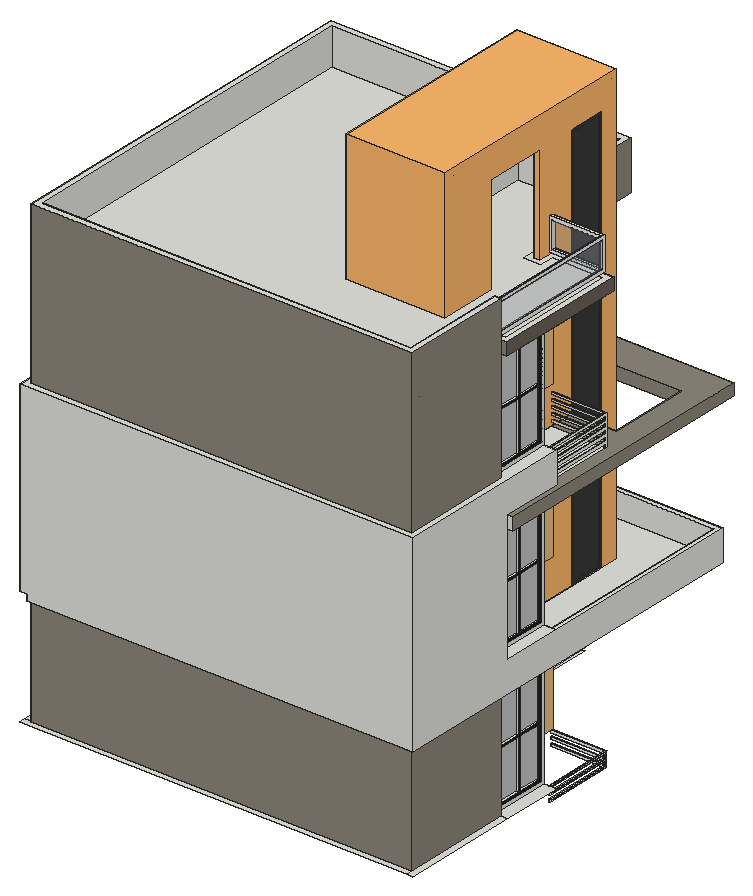
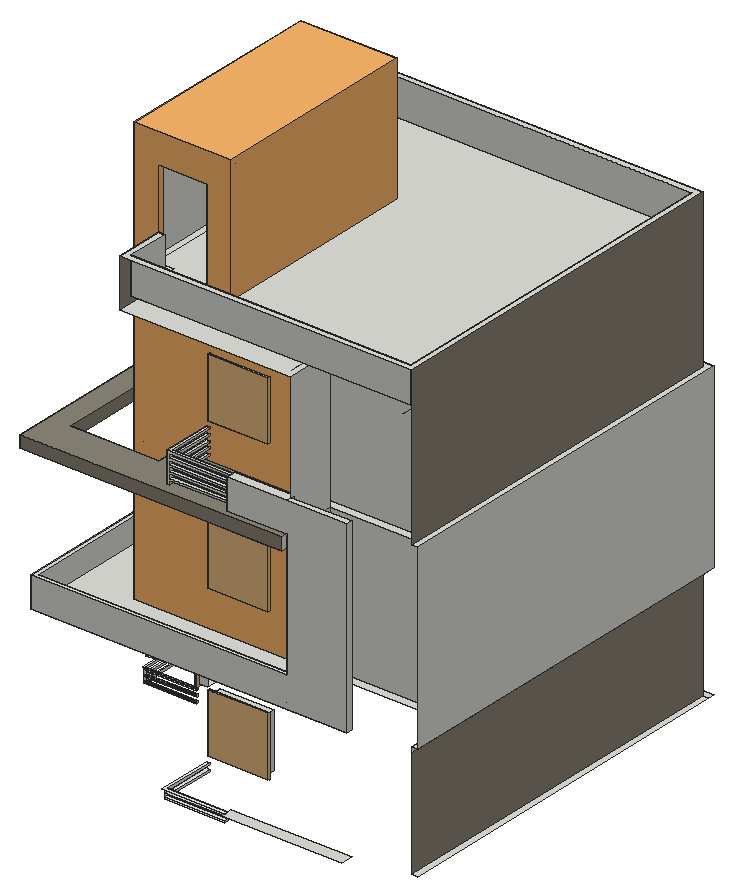
# SketchUp Ruby script. Lengths in inches.
U = 1.inch
M = Sketchup.active_model
def pt(a) = Geom::Point3d.new(a.map { |v| v * U })
def face(e, loops, mat)
  f = e.add_face(loops[0].map { |a| pt(a) })
  loops[1..].each { |l| e.add_face(l.map { |a| pt(a) }).erase! }
  f.material = f.back_material = mat if mat
  f
end
# faces: each face lists its corners as indices into pts; further lists are holes
def faces(e, pts, list, mat = nil) = list.each { |f| face(e, (f[0].is_a?(Array) ? f : [f]).map { |l| l.map { |i| pts[i] } }, mat) }
# xy, xz, yz: faces in a plane at the given z, y or x. An outline is a flat list of corners, or four numbers for a rectangle; further outlines are holes
def ring(l) = l.size == 4 ? [[l[0], l[1]], [l[2], l[1]], [l[2], l[3]], [l[0], l[3]]] : l.each_slice(2).to_a
def flat(e, list, mat, &to3) = list.each { |f| face(e, (f[0].is_a?(Array) ? f : [f]).map { |l| ring(l).map { |u, v| to3.(u, v) } }, mat) }
def xy(e, z, list, mat = nil) = flat(e, list, mat) { |x, y| [x, y, z] }
def xz(e, y, list, mat = nil) = flat(e, list, mat) { |x, z| [x, y, z] }
def yz(e, x, list, mat = nil) = flat(e, list, mat) { |y, z| [x, y, z] }
def lines(e, pts, list) = list.each { |a, b| e.add_line(pt(pts[a]), pt(pts[b])) }
# prism: a flat outline (further loops are holes) pulled along v
def prism(e, loops, v, mat = nil)
  f = face(e, loops, mat); d = Geom::Vector3d.new(v.map { |x| x * U })
  f.pushpull(f.normal.samedirection?(d) ? d.length : -d.length)
end
def box(e, o, s, mat = nil) = prism(e, [[o, [o[0] + s[0], o[1], o[2]], [o[0] + s[0], o[1] + s[1], o[2]], [o[0], o[1] + s[1], o[2]]]], [0, 0, s[2]], mat)
def at(x, y, z, deg = 0) = Geom::Transformation.translation(pt([x, y, z])) * Geom::Transformation.rotation(ORIGIN, Z_AXIS, deg.degrees)
def axes(o, x, y, z) = Geom::Transformation.new([*x, 0, *y, 0, *z, 0, *pt(o).to_a, 1])
def part(name) = M.definitions.add(name)
# library, detail: a bought-in or finely detailed component or shape, given as its bounding box
def library(name, o, s) = part(name).tap { |d| box(d.entities, o, s) }
def detail(e, o, s) = box(e.add_group.entities, o, s)
def put(e, d, t, mat = nil) = e.add_instance(d, t).tap { |i| i.material = mat if mat }
def group(e, t, mat = nil) = e.add_group.tap { |g| g.transformation = t; g.material = mat if mat }.entities
root = M.entities
M.materials.add("Brick_05_1K").color = [255, 185, 107]
M.materials.add("Glass_Basic_01").color = [161, 173, 186]
M.materials["Glass_Basic_01"].alpha = 0.25
M.materials.add("M02_Ash_Whisper").color = [196, 196, 196]
M.materials.add("M07_Charcoal_Gleam").color = [58, 58, 58]
M.materials.add("M08_Obsidian_Black").color = [30, 30, 30]
M.materials.add("Metal_06_1K").color = [238, 236, 231]
M.materials.add("Plaster_04_1K").color = [106, 98, 87]
M.materials.add("Plaster_06_1K").color = [141, 135, 122]
c1 = library("mesh-164",[-1582.71,-3144.16,-23.22],[2366.42,2227.34,65.81])
c2 = part("Group13")
put(c2.entities,c1,at(294.66,859.51,3.5))
xy(root,334,[[491.43,250.15,492.93,317.65],[438.93,317.65,491.43,319.15],[363.93,397.15,366.93,449.15],[303.93,449.15,363.93,453.15]])
xy(root,336,[[491.43,250.15,492.93,317.65],[438.93,317.65,491.43,319.15],[363.93,397.15,366.93,449.15],[303.93,449.15,363.93,453.15]],"Metal_06_1K")
xy(root,340,[[491.43,250.15,492.93,317.65],[438.93,317.65,491.43,319.15],[363.93,397.15,366.93,449.15],[303.93,449.15,363.93,453.15]])
xy(root,342,[[183.93,445.15,303.93,457.15]])
xy(root,342,[[491.43,250.15,492.93,317.65],[438.93,317.65,491.43,319.15],[363.93,397.15,366.93,397.15,366.93,453.15,303.93,453.15,303.93,449.15,363.93,449.15]],"Metal_06_1K")
xy(root,346,[[491.43,250.15,492.93,317.65],[438.93,317.65,491.43,319.15]])
xy(root,348,[[117.93,76.15,492.93,82.15],[492.93,76.15,498.93,190.15],[117.93,82.15,123.93,445.15],[482.43,190.15,486.93,250.15],[486.93,190.15,498.93,250.15]])
xy(root,348,[[491.43,250.15,492.93,250.15,492.93,319.15,438.93,319.15,438.93,317.65,491.43,317.65]],"Metal_06_1K")
xy(root,351,[[429.93,262.15,438.93,316.15],[306.93,388.15,360.93,397.15]])
xy(root,354,[[484.46,196.15,486.93,219.15],[484.46,221.15,486.93,244.15]])
xy(root,402,[[484.46,196.15,486.93,219.15],[484.46,221.15,486.93,244.15]])
xy(root,404,[[484.46,196.15,486.93,219.15],[484.46,221.15,486.93,244.15]])
xy(root,405,[[429.93,262.15,438.93,316.15],[429.93,346.15,438.93,382.15],[306.93,388.15,360.93,397.15]])
xy(root,450,[[484.46,196.15,486.93,219.15],[484.46,221.15,486.93,244.15]])
xy(root,456,[[123.93,76.15,132.93,82.15],[132.93,76.15,429.93,82.15],[492.93,76.15,492.93,190.15,486.93,190.15,486.93,250.15,482.43,250.15,482.43,190.15,438.93,190.15,438.93,397.15,243.93,397.15,243.93,445.15,183.93,445.15,183.93,451.15,498.93,451.15,498.93,76.15],[429.93,76.15,486.93,82.15],[486.93,76.15,492.93,82.15],
  [123.93,82.15,132.93,388.15],[132.93,82.15,429.93,91.15],[429.93,82.15,486.93,82.15,486.93,190.15,438.93,190.15,438.93,388.15,429.93,388.15],[486.93,82.15,492.93,190.15],[132.93,91.15,429.93,388.15]])
xy(root,462,[[117.93,76.15,123.93,445.15],[132.93,91.15,429.93,388.15],[438.93,190.15,482.43,190.15,482.43,250.15,494.43,250.15,494.43,446.65,243.93,446.65,243.93,397.15,438.93,397.15]])
xy(root,464,[[436.93,345.15,438.93,373.15],[436.93,373.15,438.93,377.15]],"M07_Charcoal_Gleam")
xy(root,486,[[482.43,190.15,486.93,250.15],[486.93,190.15,498.93,250.15],[494.43,250.15,498.93,250.15,498.93,451.15,243.93,451.15,243.93,446.65,494.43,446.65]])
xy(root,492,[[484.46,196.15,486.93,219.15],[484.46,221.15,486.93,244.15]])
xy(root,501,[[429.93,262.15,438.93,316.15],[306.93,388.15,360.93,397.15]])
xy(root,543,[[484.46,196.15,486.93,219.15],[484.46,221.15,486.93,244.15]])
xy(root,545,[[484.46,196.15,486.93,219.15],[484.46,221.15,486.93,244.15]])
xy(root,555,[[429.93,262.15,438.93,316.15],[306.93,388.15,360.93,397.15]])
xy(root,594,[[484.46,196.15,486.93,219.15],[484.46,221.15,486.93,244.15]])
xy(root,600,[[438.93,190.15,438.93,343.15,482.43,343.15,482.43,421.55,394.65,421.55,394.65,397.15,243.93,397.15,243.93,457.15,504.93,457.15,504.93,190.15,486.93,190.15,486.93,250.15,482.43,250.15,482.43,190.15]],"Plaster_06_1K")
xy(root,606,[[132.93,91.15,429.93,388.15]])
xy(root,612,[[132.93,91.15,429.93,388.15],[438.93,190.15,482.43,190.15,482.43,250.15,491.43,250.15,491.43,317.65,438.93,317.65],[486.93,190.15,498.93,250.15],[491.43,317.65,492.93,319.15],[243.93,440.65,303.93,451.15]])
xy(root,612,[[498.93,190.15,504.93,190.15,504.93,457.15,243.93,457.15,243.93,451.15,303.93,451.15,303.93,440.65,243.93,440.65,243.93,397.15,394.65,397.15,394.65,421.55,482.43,421.55,482.43,343.15,438.93,343.15,438.93,317.65,491.43,317.65,491.43,319.15,492.93,319.15,492.93,317.65,491.43,317.65,491.43,250.15,498.93,250.15]],"Plaster_06_1K")
xy(root,616,[[491.43,250.15,492.93,317.65],[438.93,317.65,491.43,319.15]])
xy(root,618,[[491.43,250.15,492.93,317.65],[438.93,317.65,491.43,319.15],[363.93,391.1,366.93,397.15],[363.93,397.15,366.93,443.15],[303.93,443.15,363.93,447.15]])
xy(root,622,[[491.43,250.15,492.93,317.65],[438.93,317.65,491.43,319.15]])
xy(root,624,[[491.43,250.15,492.93,317.65],[438.93,317.65,491.43,319.15],[363.93,391.1,366.93,397.15],[363.93,397.15,366.93,443.15],[303.93,443.15,363.93,447.15]])
xy(root,628,[[491.43,250.15,492.93,317.65],[438.93,317.65,491.43,319.15]])
xy(root,630,[[491.43,250.15,492.93,317.65],[438.93,317.65,491.43,319.15],[363.93,391.1,366.93,397.15],[363.93,397.15,366.93,443.15],[303.93,443.15,363.93,447.15]])
xy(root,634,[[491.43,250.15,492.93,317.65],[438.93,317.65,491.43,319.15]])
xy(root,636,[[491.43,250.15,492.93,317.65],[438.93,317.65,491.43,319.15],[363.93,391.15,366.93,397.15],[363.93,397.15,366.93,443.15],[303.93,443.15,363.93,447.15]])
xy(root,640,[[491.43,250.15,492.93,317.65],[438.93,317.65,491.43,319.15]])
xy(root,642,[[117.93,76.15,498.93,76.15,498.93,250.15,486.93,250.15,486.93,190.15,492.93,190.15,492.93,82.15,123.93,82.15,123.93,445.15,117.93,445.15],[486.93,82.15,492.93,190.15],[491.43,250.15,492.93,250.15,492.93,319.15,438.93,319.15,438.93,317.65,491.43,317.65],[363.93,391.15,366.93,397.15],[363.93,397.15,366.93,397.15,366.93,447.15,303.93,447.15,303.93,443.15,363.93,443.15],
  [243.93,440.65,303.93,451.15],[183.93,445.15,243.93,451.15]])
xy(root,648,[[484.46,196.15,486.93,219.15],[484.46,221.15,486.93,244.15]])
xy(root,651,[[429.93,262.15,438.93,316.15]])
xy(root,651,[[306.93,388.15,360.93,397.15]],"Brick_05_1K")
xy(root,696,[[484.46,196.15,486.93,219.15],[484.46,221.15,486.93,244.15]])
xy(root,698,[[484.46,196.15,486.93,219.15],[484.46,221.15,486.93,244.15]])
xy(root,705,[[429.93,262.15,438.93,316.15]])
xy(root,705,[[306.93,388.15,360.93,397.15]],"Brick_05_1K")
xy(root,744,[[484.46,196.15,486.93,219.15],[484.46,221.15,486.93,244.15]])
xy(root,750,[[438.93,190.15,438.93,319.15,498.93,319.15,498.93,250.15,482.43,250.15,482.43,190.15],[486.93,190.15,498.93,250.15],[243.93,397.15,414.93,445.15]])
xy(root,756,[[132.93,91.15,429.93,388.15]])
xy(root,762,[[[129.93,88.15,486.93,88.15,486.93,196.15,492.93,196.15,492.93,313.15,444.93,313.15,444.93,299.15,426.93,299.15,426.93,385.15,408.93,385.15,408.93,439.15,129.93,439.15],[342.93,190.15,342.93,397.15,366.93,397.15,366.93,391.15,348.93,391.15,348.93,199.75,432.93,199.75,432.93,245.15,438.93,245.15,438.93,190.15]],[486.93,190.15,498.93,190.15,498.93,319.15,438.93,319.15,438.93,305.15,432.93,305.15,432.93,391.15,414.93,391.15,414.93,397.15,408.93,397.15,408.93,385.15,426.93,385.15,426.93,299.15,444.93,299.15,444.93,313.15,492.93,313.15,492.93,196.15,486.93,196.15]])
xy(root,764,[[488.93,190.15,488.93,316.15,438.93,316.15,438.93,319.15,490.93,319.15,490.93,190.15]])
xy(root,767,[[488.93,193.15,490.93,316.15],[441.93,316.15,487.93,319.15]])
xy(root,793,[[488.93,193.15,490.93,316.15],[441.93,316.15,487.93,319.15]])
xy(root,796,[[488.93,190.15,490.93,190.15,490.93,319.15,438.93,319.15,438.93,316.15,488.93,316.15]],"Metal_06_1K")
xy(root,798,[[123.93,82.15,492.93,82.15,492.93,190.15,486.93,190.15,486.93,88.15,129.93,88.15,129.93,439.15,408.93,439.15,408.93,397.15,414.93,397.15,414.93,445.15,123.93,445.15]])
xy(root,856,[[436.93,345.15,438.93,377.15]],"M07_Charcoal_Gleam")
xy(root,858,[[432.93,245.15,438.93,305.15],[366.93,391.15,414.93,397.15]],"Brick_05_1K")
xy(root,882,[[348.93,199.75,432.93,391.15]])
xy(root,888,[[342.93,190.15,438.93,397.15]],"Brick_05_1K")
xz(root,76.15,[[123.93,456,498.93,456,498.93,642,117.93,642,117.93,462,123.93,462]])
xz(root,82.15,[[123.93,348,492.93,456],[123.93,642,492.93,798]],"Plaster_06_1K")
xz(root,88.15,[[129.93,762,486.93,798]])
xz(root,91.15,[[132.93,462,429.93,606],[132.93,612,429.93,756]])
xz(root,190.15,[[482.43,348,486.93,456],[486.93,348,492.93,456],[438.93,462,482.43,600],[486.93,486,498.93,600],[486.93,600,498.93,612],
  [498.93,600,504.93,612],[438.93,612,482.43,750],[486.93,642,492.93,750],[[486.93,762,492.93,798],[488.93,764,490.93,796]]])
xz(root,190.15,[[342.93,762,438.93,888]],"Brick_05_1K")
xz(root,190.15,[[492.93,750,498.93,762]],"Plaster_06_1K")
xz(root,193.15,[[488.93,767,490.93,793]])
xz(root,196.15,[[484.46,354,486.93,402],[484.46,404,486.93,450],[484.46,492,486.93,543],[484.46,545,486.93,594],[484.46,648,486.93,696],
  [484.46,698,486.93,744]])
xz(root,199.75,[[348.93,762,432.93,882]])
xz(root,219.15,[[484.46,354,486.93,402],[484.46,404,486.93,450],[484.46,492,486.93,543],[484.46,545,486.93,594],[484.46,648,486.93,696],
  [484.46,698,486.93,744]])
xz(root,221.15,[[484.46,354,486.93,402],[484.46,404,486.93,450],[484.46,492,486.93,543],[484.46,545,486.93,594],[484.46,648,486.93,696],
  [484.46,698,486.93,744]])
xz(root,244.15,[[484.46,354,486.93,402],[484.46,404,486.93,450],[484.46,492,486.93,543],[484.46,545,486.93,594],[484.46,648,486.93,696],
  [484.46,698,486.93,744]])
xz(root,245.15,[[432.93,762,438.93,858]],"Brick_05_1K")
xz(root,250.15,[[491.43,334,492.93,336],[491.43,340,492.93,342],[491.43,346,492.93,348],[482.43,348,486.93,456],[482.43,462,486.93,486],
  [486.93,462,494.43,486],[482.43,486,486.93,600],[[482.43,612,482.43,642,491.43,642,491.43,640,492.93,640,492.93,642,498.93,642,498.93,612],[491.43,616,492.93,618],[491.43,622,492.93,624],[491.43,628,492.93,630],[491.43,634,492.93,636]],[482.43,642,486.93,750]])
xz(root,262.15,[[429.93,351,438.93,405],[429.93,501,438.93,555],[429.93,651,438.93,705]])
xz(root,305.15,[[432.93,762,438.93,858]],"Brick_05_1K")
xz(root,316.15,[[429.93,351,438.93,405],[429.93,501,438.93,555],[429.93,651,438.93,705],[488.93,767,490.93,793]])
xz(root,316.15,[[[438.93,764,488.93,796],[441.93,767,487.93,793]]],"Metal_06_1K")
xz(root,317.65,[[491.43,336,492.93,340],[491.43,342,492.93,346],[491.43,612,492.93,614],[491.43,614,492.93,616],[438.93,616,491.43,618],
  [491.43,618,492.93,620],[491.43,620,492.93,622],[438.93,622,491.43,624],[491.43,624,492.93,626],[491.43,626,492.93,628],
  [438.93,628,491.43,630],[491.43,630,492.93,632],[491.43,632,492.93,634],[438.93,634,491.43,636],[491.43,636,492.93,638],
  [491.43,638,492.93,640],[438.93,640,491.43,642]])
xz(root,317.65,[[438.93,334,491.43,336],[438.93,340,491.43,342],[438.93,346,491.43,348]],"Metal_06_1K")
xz(root,319.15,[[441.93,767,487.93,793]],"Glass_Basic_01")
xz(root,319.15,[[491.43,612,491.43,616,438.93,616,438.93,618,491.43,618,491.43,622,438.93,622,438.93,624,491.43,624,491.43,628,438.93,628,438.93,630,491.43,630,491.43,634,438.93,634,438.93,636,491.43,636,491.43,640,438.93,640,438.93,642,492.93,642,492.93,612],[[438.93,764,490.93,796],[441.93,767,487.93,793]]],"Metal_06_1K")
xz(root,319.15,[[438.93,750,498.93,762]],"Plaster_04_1K")
xz(root,343.15,[[438.93,600,482.43,612]],"Plaster_06_1K")
xz(root,345.15,[[436.93,464,438.93,600],[436.93,600,438.93,612],[436.93,612,438.93,856]],"M07_Charcoal_Gleam")
xz(root,377.15,[[436.93,464,438.93,856]],"M07_Charcoal_Gleam")
xz(root,388.15,[[[132.93,462,429.93,606],[306.93,501,360.93,555]],[[132.93,612,429.93,756],[306.93,651,360.93,705]]])
xz(root,391.15,[[348.93,762,366.93,762,366.93,858,414.93,858,414.93,762,432.93,762,432.93,882,348.93,882]])
xz(root,397.15,[[243.93,600,394.65,606],[243.93,750,366.93,756],[366.93,750,414.93,756],[408.93,762,414.93,798]])
xz(root,397.15,[[[303.93,348,363.93,408],[306.93,351,360.93,405]],[[243.93,462,243.93,600,394.65,600,394.65,612,243.93,612,243.93,750,414.93,750,414.93,858,366.93,858,366.93,762,342.93,762,342.93,888,438.93,888,438.93,462],[303.93,648,363.93,708],[303.93,498,363.93,558]],[[303.93,498,363.93,558],[306.93,501,360.93,555]],[[303.93,648,363.93,708],[306.93,651,360.93,705]]],"Brick_05_1K")
xz(root,421.55,[[394.65,600,482.43,612]],"Plaster_06_1K")
xz(root,439.15,[[129.93,762,408.93,798]])
xz(root,440.65,[[243.93,612,303.93,642]])
xz(root,443.15,[[363.93,612,366.93,616],[303.93,616,363.93,618],[363.93,618,366.93,622],[303.93,622,363.93,624],[363.93,624,366.93,628],
  [303.93,628,363.93,630],[363.93,630,366.93,634],[303.93,634,363.93,636],[363.93,636,366.93,640],[303.93,640,363.93,642]])
xz(root,446.65,[[243.93,462,494.43,486]])
xz(root,447.15,[[363.93,612,363.93,616,303.93,616,303.93,618,363.93,618,363.93,622,303.93,622,303.93,624,363.93,624,363.93,628,303.93,628,303.93,630,363.93,630,363.93,634,303.93,634,303.93,636,363.93,636,363.93,640,303.93,640,303.93,642,366.93,642,366.93,612]],"Metal_06_1K")
xz(root,449.15,[[303.93,334,363.93,336],[363.93,336,366.93,340],[303.93,340,363.93,342]])
xz(root,451.15,[[183.93,456,183.93,642,303.93,642,303.93,612,243.93,612,243.93,486,498.93,486,498.93,456]])
xz(root,457.15,[[243.93,600,504.93,612]],"Plaster_06_1K")
yz(root,117.93,[[76.15,462,445.15,642]])
yz(root,123.93,[[76.15,456,445.15,462]])
yz(root,123.93,[[82.15,348,445.15,456],[82.15,642,445.15,798]],"Plaster_06_1K")
yz(root,129.93,[[88.15,762,439.15,798]])
yz(root,132.93,[[91.15,462,388.15,606],[91.15,612,388.15,756]])
yz(root,183.93,[[445.15,456,451.15,642]])
yz(root,243.93,[[397.15,462,446.65,462,446.65,486,451.15,486,451.15,600,397.15,600],[397.15,600,451.15,612],[451.15,600,457.15,612],[397.15,612,440.65,612,440.65,642,445.15,642,445.15,750,397.15,750]])
yz(root,303.93,[[449.15,334,453.15,336],[449.15,340,453.15,342],[440.65,612,451.15,642]])
yz(root,306.93,[[388.15,351,397.15,405],[388.15,501,397.15,555]])
yz(root,306.93,[[388.15,651,397.15,705]],"Brick_05_1K")
yz(root,342.93,[[190.15,762,397.15,888]],"Brick_05_1K")
yz(root,348.93,[[199.75,762,391.15,882]])
yz(root,360.93,[[388.15,351,397.15,405],[388.15,501,397.15,555]])
yz(root,360.93,[[388.15,651,397.15,705]],"Brick_05_1K")
yz(root,363.93,[[449.15,336,453.15,340],[443.15,612,447.15,616],[391.1,616,397.15,618],[397.15,616,443.15,618],[443.15,618,447.15,622],
  [391.1,622,397.15,624],[397.15,622,443.15,624],[443.15,624,447.15,628],[391.1,628,397.15,630],[397.15,628,443.15,630],
  [443.15,630,447.15,634],[391.15,634,397.15,636],[397.15,634,443.15,636],[443.15,636,447.15,640],[391.15,640,397.15,642],
  [397.15,640,443.15,642]])
yz(root,363.93,[[397.15,334,449.15,336],[397.15,340,449.15,342]],"Metal_06_1K")
yz(root,366.93,[[391.1,616,397.15,618],[391.1,622,397.15,624],[391.1,628,397.15,630],[391.15,634,397.15,636],[391.15,640,397.15,642]])
yz(root,366.93,[[391.15,762,397.15,858]],"Brick_05_1K")
yz(root,366.93,[[443.15,612,447.15,612,447.15,642,397.15,642,397.15,640,443.15,640,443.15,636,397.15,636,397.15,634,443.15,634,443.15,630,397.15,630,397.15,628,443.15,628,443.15,624,397.15,624,397.15,622,443.15,622,443.15,618,397.15,618,397.15,616,443.15,616]],"Metal_06_1K")
yz(root,394.65,[[397.15,600,421.55,612]],"Plaster_06_1K")
yz(root,408.93,[[397.15,762,439.15,798]])
yz(root,414.93,[[391.15,762,397.15,858]],"Brick_05_1K")
yz(root,414.93,[[397.15,750,445.15,798]],"Plaster_06_1K")
yz(root,429.93,[[[91.15,462,388.15,606],[262.15,501,316.15,555]],[[91.15,612,388.15,756],[262.15,651,316.15,705]]])
yz(root,432.93,[[199.75,762,199.75,882,391.15,882,391.15,762,305.15,762,305.15,858,245.15,858,245.15,762]])
yz(root,436.93,[[345.15,464,377.15,856]],"M07_Charcoal_Gleam")
yz(root,438.93,[[317.65,334,319.15,336],[317.65,340,319.15,342],[[259.15,348,319.15,408],[262.15,351,316.15,405]],[190.15,456,343.15,462],[343.15,456,373.15,462],
  [373.15,456,379.15,462],[[259.15,498,319.15,558],[262.15,501,316.15,555]],[190.15,600,343.15,612],[[259.15,648,319.15,708],[262.15,651,316.15,705]]])
yz(root,438.93,[[[190.15,462,343.15,600],[259.15,498,319.15,558]],[[379.15,462,397.15,462,397.15,888,190.15,888,190.15,762,245.15,762,245.15,858,305.15,858,305.15,762,319.15,762,319.15,750,190.15,750,190.15,612,343.15,612,343.15,858,379.15,858],[259.15,648,319.15,708],[316.15,764,319.15,796],[317.65,616,319.15,618],[317.65,622,319.15,624],[317.65,634,319.15,636],[317.65,640,319.15,642],[317.65,628,319.15,630]]],"Brick_05_1K")
yz(root,438.93,[[[343.15,462,379.15,858],[345.15,464,377.15,856]]],"M07_Charcoal_Gleam")
yz(root,441.93,[[316.15,767,319.15,793]])
yz(root,482.43,[[190.15,348,250.15,456],[190.15,462,194.65,486],[194.65,462,250.15,486],[190.15,486,250.15,600],[190.15,612,250.15,618],
  [190.15,618,250.15,750]])
yz(root,482.43,[[343.15,600,421.55,612]],"Plaster_06_1K")
yz(root,484.46,[[196.15,354,219.15,402],[221.15,354,244.15,402],[196.15,404,219.15,450],[221.15,404,244.15,450],[196.15,492,219.15,543],
  [221.15,492,244.15,543],[196.15,545,219.15,594],[221.15,545,244.15,594],[196.15,648,219.15,696],[221.15,648,244.15,696],
  [196.15,698,219.15,744],[221.15,698,244.15,744]],"M02_Ash_Whisper")
yz(root,486.93,[[[190.15,348,250.15,456],[193.15,351,247.15,453]],[193.15,456,247.15,459],[[190.15,486,250.15,600],[193.15,489,247.15,597]],[[190.15,642,250.15,750],[193.15,645,247.15,747]],[88.15,762,190.15,798]])
yz(root,486.93,[[193.15,351,247.15,351,247.15,453,244.15,453,244.15,354,196.15,354,196.15,453,193.15,453],[219.15,354,221.15,354,221.15,402,244.15,402,244.15,404,221.15,404,221.15,450,219.15,450,219.15,404,196.15,404,196.15,402,219.15,402],[196.15,450,244.15,453],[[193.15,489,247.15,597],[196.15,492,244.15,594]],[219.15,492,221.15,492,221.15,543,244.15,543,244.15,545,221.15,545,221.15,594,219.15,594,219.15,545,196.15,545,196.15,543,219.15,543],
  [[193.15,645,247.15,747],[196.15,648,244.15,744]],[219.15,648,221.15,648,221.15,696,244.15,696,244.15,698,221.15,698,221.15,744,219.15,744,219.15,698,196.15,698,196.15,696,219.15,696]],"M08_Obsidian_Black")
yz(root,487.93,[[316.15,767,319.15,793]])
yz(root,488.93,[[190.15,764,190.15,796,316.15,796,316.15,793,193.15,793,193.15,767,316.15,767,316.15,764]],"Metal_06_1K")
yz(root,490.93,[[193.15,767,316.15,793]],"Glass_Basic_01")
yz(root,490.93,[[[190.15,764,319.15,796],[193.15,767,316.15,793]]],"Metal_06_1K")
yz(root,491.43,[[250.15,334,317.65,336],[317.65,336,319.15,340],[250.15,340,317.65,342],[317.65,342,319.15,346],[250.15,346,317.65,348],
  [317.65,612,319.15,614],[317.65,614,319.15,616],[250.15,616,317.65,618],[317.65,618,319.15,620],[317.65,620,319.15,622],
  [250.15,622,317.65,624],[317.65,624,319.15,626],[317.65,626,319.15,628],[250.15,628,317.65,630],[317.65,630,319.15,632],
  [317.65,632,319.15,634],[250.15,634,317.65,636],[317.65,636,319.15,638],[317.65,638,319.15,640],[250.15,640,317.65,642]])
yz(root,492.93,[[317.65,612,319.15,612,319.15,642,250.15,642,250.15,640,317.65,640,317.65,636,250.15,636,250.15,634,317.65,634,317.65,630,250.15,630,250.15,628,317.65,628,317.65,624,250.15,624,250.15,622,317.65,622,317.65,618,250.15,618,250.15,616,317.65,616]],"Metal_06_1K")
yz(root,492.93,[[82.15,348,190.15,456],[82.15,642,190.15,798]],"Plaster_06_1K")
yz(root,494.43,[[250.15,462,446.65,486]])
yz(root,498.93,[[76.15,456,451.15,456,451.15,486,190.15,486,190.15,612,250.15,612,250.15,642,76.15,642]])
yz(root,498.93,[[190.15,750,319.15,762]],"Plaster_04_1K")
yz(root,504.93,[[190.15,600,457.15,612]],"Plaster_06_1K")
p = [[429.93,388.15,606],[429.93,397.15,606],[132.93,388.15,606],[123.93,388.15,606],[132.93,91.15,606],[132.93,82.15,606],
  [429.93,91.15,756],[492.93,91.15,756],[429.93,388.15,756],[429.93,397.15,756],[132.93,388.15,756],[132.93,445.15,756],
  [243.93,397.15,456],[243.93,397.15,462],[243.93,397.15,756],[243.93,445.15,756],[482.43,190.15,462],[486.93,190.15,462],
  [248.43,440.65,462],[243.93,440.65,462],[482.43,190.15,618],[486.93,190.15,618],[486.93,250.15,456],[486.93,250.15,462],
  [482.43,190.15,606],[482.43,190.15,600],[486.93,247.15,753],[486.93,193.15,753],[486.93,193.15,750],[486.93,247.15,750],
  [366.93,397.15,616],[366.93,397.15,615.9375],[363.93,397.15,634],[363.93,397.15,633.83],[243.93,446.65,462],[243.93,451.15,462],
  [348.93,391.15,882],[342.93,391.15,882],[432.93,199.75,882],[438.93,199.75,882],[432.93,391.15,882],[438.93,391.15,882]]
lines(root,p,[[0,1],[2,3],[4,5],[6,7],[8,9],[10,11],[12,13],[14,15],[16,17],[18,19],[20,21],[22,23],
  [24,25],[26,27],[27,28],[29,26],[30,31],[32,33],[34,35],[36,37],[38,39],[40,41]])
put(root,c2,axes([440.09,286.51,409.53],[0,-0.02533,0],[0,0,0.02667],[-0.02533,0,0]))
put(root,c2,axes([336.56,398.3125,409.53],[0.02533,0,0],[0,0,0.02667],[0,-0.02533,0]))
put(root,c2,axes([440.09,286.51,559.53],[0,-0.02533,0],[0,0,0.02667],[-0.02533,0,0]))
put(root,c2,axes([336.56,398.3125,559.53],[0.02533,0,0],[0,0,0.02667],[0,-0.02533,0]))
put(root,c2,axes([440.09,286.51,709.53],[0,-0.02533,0],[0,0,0.02667],[-0.02533,0,0]))
put(root,c2,axes([336.56,398.3125,709.53],[0.02533,0,0],[0,0,0.02667],[0,-0.02533,0]))
